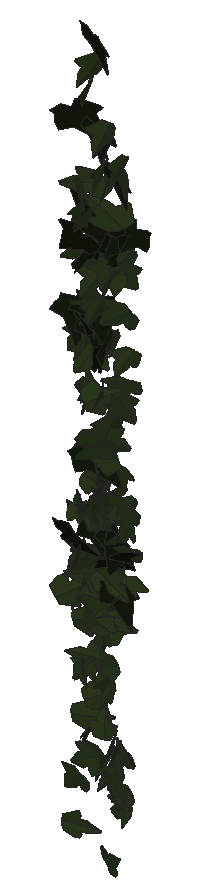
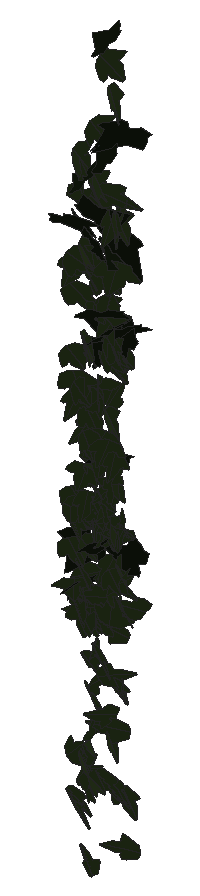
# SketchUp Ruby script. Lengths in inches.
U = 1.inch
M = Sketchup.active_model
def pt(a) = Geom::Point3d.new(a.map { |v| v * U })
def face(e, loops, mat)
  f = e.add_face(loops[0].map { |a| pt(a) })
  loops[1..].each { |l| e.add_face(l.map { |a| pt(a) }).erase! }
  f.material = f.back_material = mat if mat
  f
end
# faces: each face lists its corners as indices into pts; further lists are holes
def faces(e, pts, list, mat = nil) = list.each { |f| face(e, (f[0].is_a?(Array) ? f : [f]).map { |l| l.map { |i| pts[i] } }, mat) }
# xy, xz, yz: faces in a plane at the given z, y or x. An outline is a flat list of corners, or four numbers for a rectangle; further outlines are holes
def ring(l) = l.size == 4 ? [[l[0], l[1]], [l[2], l[1]], [l[2], l[3]], [l[0], l[3]]] : l.each_slice(2).to_a
def flat(e, list, mat, &to3) = list.each { |f| face(e, (f[0].is_a?(Array) ? f : [f]).map { |l| ring(l).map { |u, v| to3.(u, v) } }, mat) }
def xy(e, z, list, mat = nil) = flat(e, list, mat) { |x, y| [x, y, z] }
def xz(e, y, list, mat = nil) = flat(e, list, mat) { |x, z| [x, y, z] }
def yz(e, x, list, mat = nil) = flat(e, list, mat) { |y, z| [x, y, z] }
def lines(e, pts, list) = list.each { |a, b| e.add_line(pt(pts[a]), pt(pts[b])) }
# prism: a flat outline (further loops are holes) pulled along v
def prism(e, loops, v, mat = nil)
  f = face(e, loops, mat); d = Geom::Vector3d.new(v.map { |x| x * U })
  f.pushpull(f.normal.samedirection?(d) ? d.length : -d.length)
end
def box(e, o, s, mat = nil) = prism(e, [[o, [o[0] + s[0], o[1], o[2]], [o[0] + s[0], o[1] + s[1], o[2]], [o[0], o[1] + s[1], o[2]]]], [0, 0, s[2]], mat)
def at(x, y, z, deg = 0) = Geom::Transformation.translation(pt([x, y, z])) * Geom::Transformation.rotation(ORIGIN, Z_AXIS, deg.degrees)
def axes(o, x, y, z) = Geom::Transformation.new([*x, 0, *y, 0, *z, 0, *pt(o).to_a, 1])
def part(name) = M.definitions.add(name)
# library, detail: a bought-in or finely detailed component or shape, given as its bounding box
def library(name, o, s) = part(name).tap { |d| box(d.entities, o, s) }
def detail(e, o, s) = box(e.add_group.entities, o, s)
def put(e, d, t, mat = nil) = e.add_instance(d, t).tap { |i| i.material = mat if mat }
def group(e, t, mat = nil) = e.add_group.tap { |g| g.transformation = t; g.material = mat if mat }.entities
root = M.entities
M.materials.add("1026 AP 7946 SUNNY SIDE UP").color = [254, 231, 186]
M.materials.add("efeu1").color = [18, 25, 13]
M.materials.add("efeu2").color = [43, 57, 29]
c1 = part("ivyleaf_10")
p = [[0,0.5,-0.03],[-0.0625,2.02,-0.43],[-0.19,2.01,-0.46],[-0.54,1.05,-0.29],[-0.52,0.625,-0.18],[-0.83,0.76,-0.28],
  [-1.16,0.64,-0.33],[-1.15,0.33,-0.24],[-0.77,-0.39,0.02],[-0.3,-0.51,0.16],[0.04,-0.48,0.23],[-0.02,2.01,-0.4375],
  [-0.06,2.01,-0.43],[0.04,-0.49,0.23],[0.67,-0.49,0.14],[1.38,0.36,-0.2],[1.375,0.51,-0.24],[0.81,0.65,-0.19],
  [0.62,0.59,-0.15],[0.6,1.09,-0.28],[0.5,1.23,-0.31]]
faces(c1.entities,p,[[0,1,2,3,4,5,6,7,8,9,10],[11,12,0,13,14,15,16,17,18,19,20]],"efeu2")
c2 = part("ivyleaf_9")
p = [[1.54,2.16,1.25],[1.36,2.04,1.19],[-0.21,0.99,0.68],[-0.71,1.11,0.82],[-0.85,0.86,0.67],[-0.8,0.17,0.21],
  [-0.9,-0.01,0.1],[-0.67,-0.16,-0.02],[-0.08,-0.08,-0.05],[-0.03,-0.6,-0.4],[0.65,-0.88,-0.66],[0.83,-0.6,-0.49],
  [1.29,-0.42,-0.43],[1.8125,-0.07,-0.26],[1.21,0.44,0.15]]
faces(c2.entities,p,[[0,1,2,3,4,5,6,7,8,9,10,11,12,13,14]],"efeu1")
put(root,c1,axes([103.61,212.21,251.89],[-0.27089,0.03571,0.13207],[-0.20428,-0.00122,-0.1798],[-0.04391,-0.21462,0.02171]),"1026 AP 7946 SUNNY SIDE UP")
put(root,c1,axes([103.41,212.46,256.41],[-0.01976,-0.0299,0.20715],[0.11354,-0.18916,-0.02541],[0.29909,0.06983,0.02333]),"1026 AP 7946 SUNNY SIDE UP")
put(root,c2,axes([103.42,212.48,261.66],[-0.15715,-0.22456,-0.02631],[0.03236,0.01737,-0.25284],[0.35368,-0.10137,0.01144]),"1026 AP 7946 SUNNY SIDE UP")
put(root,c2,axes([103.32,212.4375,265.83],[-0.04557,-0.10489,-0.2458],[0.10836,0.22782,-0.11074],[0.39435,-0.07472,0.00202]),"1026 AP 7946 SUNNY SIDE UP")
put(root,c1,axes([103.59,212.45,261.22],[-0.1334,-0.17505,0.12633],[-0.05609,-0.11957,-0.20034],[0.33227,-0.09047,0.0169]),"1026 AP 7946 SUNNY SIDE UP")
put(root,c1,axes([103.43,212.65,258.53],[0.02494,-0.08582,0.20176],[0.14177,-0.17592,-0.08775],[0.30564,0.08861,0.02424]),"1026 AP 7946 SUNNY SIDE UP")
put(root,c2,axes([103.7,212.21,263.39],[0.16186,0.04053,-0.2429],[-0.35017,-0.07823,-0.11436],[-0.13841,0.24531,0.00528]),"1026 AP 7946 SUNNY SIDE UP")
put(root,c2,axes([103.22,212.32,256.83],[0.1703,-0.08723,0.20732],[0.20863,-0.15336,-0.14259],[0.27553,0.17004,-0.02018]),"1026 AP 7946 SUNNY SIDE UP")
put(root,c1,axes([103.45,212.41,255.82],[0.21725,-0.13904,0.11243],[0.10022,-0.09107,-0.20175],[0.26006,0.15125,-0.01617]),"1026 AP 7946 SUNNY SIDE UP")
put(root,c1,axes([103.5625,212.41,263.875],[0.01779,-0.23922,0.05053],[0.00255,-0.05039,-0.24701],[0.3844,0.0114,-0.0007]),"1026 AP 7946 SUNNY SIDE UP")
put(root,c1,axes([103.33,212.11,255.72],[0.14201,0.05417,-0.23523],[0.27143,0.15089,0.10795],[0.25066,-0.19408,0.01637]),"1026 AP 7946 SUNNY SIDE UP")
put(root,c1,axes([103.48,212.625,257.33],[0.0058,-0.07142,-0.19984],[0.01406,-0.19337,0.07255],[-0.32413,-0.00966,-0.00043]),"1026 AP 7946 SUNNY SIDE UP")
put(root,c1,axes([103.55,212.53,258.38],[-0.28661,0.09379,-0.01114],[0.00341,-0.0205,-0.21055],[-0.14851,-0.18147,0.01667]),"1026 AP 7946 SUNNY SIDE UP")
put(root,c1,axes([103.79,212.53,264.39],[0.16776,-0.0179,-0.23952],[-0.36435,-0.03577,-0.10696],[-0.03961,0.2532,-0.03052]),"1026 AP 7946 SUNNY SIDE UP")
put(root,c1,axes([103.47,212.4375,257.42],[0.18217,0.16732,0.0433],[0.0408,0.03199,-0.20945],[-0.26782,0.11869,-0.00246]),"1026 AP 7946 SUNNY SIDE UP")
put(root,c1,axes([103.71,212.49,252.23],[0.21608,-0.11136,-0.16322],[-0.21478,0.08089,-0.18087],[0.21472,0.19298,-0.01667]),"1026 AP 7946 SUNNY SIDE UP")
put(root,c1,axes([103.6,212.5625,256.54],[-0.12165,-0.17288,0.0748],[0.00088,-0.0798,-0.19298],[0.29544,-0.07094,0.03137]),"1026 AP 7946 SUNNY SIDE UP")
put(root,c1,axes([103.57,212.48,262.87],[-0.31656,-0.14651,-0.05002],[0.07939,0.01146,-0.2556],[0.2289,-0.20658,0.01948]),"1026 AP 7946 SUNNY SIDE UP")
put(root,c2,axes([103.34,212.44,261.35],[0.05466,-0.05707,0.26462],[0.13403,-0.24302,-0.06884],[0.39195,0.09106,-0.01336]),"1026 AP 7946 SUNNY SIDE UP")
put(root,c1,axes([103.83,212.31,257.33],[-0.05493,0.01768,-0.23778],[-0.29981,0.13034,0.04076],[0.20667,0.19378,-0.00407]),"1026 AP 7946 SUNNY SIDE UP")
put(root,c1,axes([103.48,212.39,264.24],[-0.13911,0.15671,-0.1847],[0.10801,-0.16733,-0.18565],[-0.35961,-0.11088,0.01569]),"1026 AP 7946 SUNNY SIDE UP")
put(root,c1,axes([103.53,212.39,256.65],[0.13148,-0.15203,0.1541],[0.09992,-0.13659,-0.17937],[0.32113,0.10475,-0.00728]),"1026 AP 7946 SUNNY SIDE UP")
put(root,c1,axes([103.41,212.44,257.58],[0.0799,-0.05103,0.19479],[0.24753,-0.10607,-0.07358],[0.18394,0.16491,0.0144]),"1026 AP 7946 SUNNY SIDE UP")
put(root,c1,axes([103.61,212.46,258.91],[-0.10047,-0.1749,-0.09713],[0.05897,0.08558,-0.19125],[0.30607,-0.0739,0.00497]),"1026 AP 7946 SUNNY SIDE UP")
put(root,c1,axes([103.63,212.59,259.85],[0.06703,-0.21488,0.03634],[0.00113,-0.03705,-0.2258],[0.34271,0.04215,-0.00636]),"1026 AP 7946 SUNNY SIDE UP")
put(root,c1,axes([103.38,212.26,250.8],[0.00055,0.01424,0.21153],[0.27157,0.11152,-0.00762],[-0.1758,0.17231,-0.01111]),"1026 AP 7946 SUNNY SIDE UP")
put(root,c1,axes([103.64,212.41,263.86],[0.19636,-0.18165,-0.1106],[-0.0115,0.11981,-0.21902],[0.33076,0.112,0.05804]),"1026 AP 7946 SUNNY SIDE UP")
put(root,c1,axes([103.67,212.5,255.59],[-0.33341,-0.03051,-0.01818],[-0.03117,0.01551,0.21999],[-0.04566,0.21219,-0.01742]),"1026 AP 7946 SUNNY SIDE UP")
put(root,c1,axes([103.79,212.48,254.35],[0.04297,0.05696,0.19953],[-0.17276,-0.15938,0.06343],[0.26573,-0.11283,0.00898]),"1026 AP 7946 SUNNY SIDE UP")
put(root,c1,axes([103.7,212.49,261.08],[-0.04657,-0.19853,0.13565],[-0.02194,-0.13215,-0.2075],[0.37493,-0.0324,0.00471]),"1026 AP 7946 SUNNY SIDE UP")
put(root,c1,axes([103.67,212.45,266.45],[0.07942,-0.2511,-0.02711],[-0.00605,0.02462,-0.26372],[0.39673,0.05064,0.0014]),"1026 AP 7946 SUNNY SIDE UP")
put(root,c1,axes([103.71,212.36,254.23],[0.26888,-0.09045,-0.06429],[-0.09491,0.018,-0.19882],[0.14384,0.18096,-0.01102]),"1026 AP 7946 SUNNY SIDE UP")
put(root,c1,axes([103.85,212.49,252.25],[0.17274,-0.10111,-0.19148],[-0.23638,0.10917,-0.15254],[0.233,0.1857,-0.01279]),"1026 AP 7946 SUNNY SIDE UP")
put(root,c1,axes([103.48,212.39,254.14],[0.10128,-0.04643,0.21667],[0.27428,-0.11799,-0.08246],[0.19935,0.18593,0.00337]),"1026 AP 7946 SUNNY SIDE UP")
put(root,c1,axes([103.9,212.28,256.24],[0.15765,-0.04672,-0.2011],[-0.30141,0.04145,-0.11155],[0.09225,0.21526,-0.0208]),"1026 AP 7946 SUNNY SIDE UP")
put(root,c1,axes([103.73,212.4375,261.38],[0.24024,-0.1706,-0.04919],[-0.0443,0.03756,-0.23567],[0.2746,0.15531,0.00501]),"1026 AP 7946 SUNNY SIDE UP")
put(root,c1,axes([103.69,212.43,260.05],[-0.04311,0.13514,0.20024],[0.08955,-0.18536,0.14052],[0.36029,0.06224,-0.01097]),"1026 AP 7946 SUNNY SIDE UP")
put(root,c1,axes([103.65,212.51,256.11],[0.01373,-0.04375,0.21633],[0.13983,-0.19079,-0.04582],[0.30735,0.08875,0.01118]),"1026 AP 7946 SUNNY SIDE UP")
put(root,c2,axes([103.87,212.15,262.97],[-0.22621,0.11335,-0.18737],[-0.19582,0.13501,0.18828],[0.2753,0.18917,-0.02004]),"1026 AP 7946 SUNNY SIDE UP")
put(root,c1,axes([103.71,212.5,261.36],[-0.01107,-0.17117,0.17476],[0.10213,-0.16574,-0.16952],[0.36603,0.04107,0.05259]),"1026 AP 7946 SUNNY SIDE UP")
put(root,c1,axes([103.9375,212.45,257.85],[-0.04535,0.04392,-0.20433],[-0.20651,0.14913,0.0545],[0.2442,0.13427,0.00814]),"1026 AP 7946 SUNNY SIDE UP")
put(root,c1,axes([103.76,212.32,263.77],[-0.07787,-0.20824,-0.14961],[0.07406,0.13663,-0.21937],[0.39118,-0.06732,0.01175]),"1026 AP 7946 SUNNY SIDE UP")
put(root,c2,axes([103.59,212.74,265.19],[0.04774,-0.17271,0.19226],[0.05207,-0.18466,-0.18174],[0.39757,0.04493,0.00072]),"1026 AP 7946 SUNNY SIDE UP")
put(root,c1,axes([103.84,212.46,261.79],[-0.32319,-0.10845,-0.05212],[-0.08072,-0.00957,0.23885],[-0.16953,0.21131,-0.01437]),"1026 AP 7946 SUNNY SIDE UP")
put(root,c1,axes([103.8125,212.37,260.9],[0.38473,-0.03452,-0.07064],[-0.11174,-0.01692,-0.25328],[0.04494,0.25349,-0.02501]),"1026 AP 7946 SUNNY SIDE UP")
put(root,c1,axes([103.83,212.3,252.99],[0.06254,-0.20851,-0.01696],[-0.01359,0.0139,-0.21851],[0.32846,0.04028,-0.00581]),"1026 AP 7946 SUNNY SIDE UP")
put(root,c1,axes([103.87,212.39,267.03],[-0.06527,-0.20567,0.16384],[-0.00571,-0.16175,-0.21584],[0.40988,-0.035,0.02308]),"1026 AP 7946 SUNNY SIDE UP")
put(root,c1,axes([103.85,212.45,257.18],[0.01619,0.2023,-0.07831],[-0.00197,0.07731,0.20907],[0.34045,-0.00917,0.00494]),"1026 AP 7946 SUNNY SIDE UP")
put(root,c1,axes([103.74,212.53,261.64],[-0.25801,0.11085,-0.11509],[0.09552,-0.10523,-0.19897],[-0.22906,-0.16874,0.04667]),"1026 AP 7946 SUNNY SIDE UP")
put(root,c1,axes([103.79,212.46,259.12],[-0.22339,-0.14035,-0.0661],[0.09909,0.02568,-0.20399],[0.22093,-0.15343,0.02465]),"1026 AP 7946 SUNNY SIDE UP")
put(root,c1,axes([103.875,212.27,257.67],[0.04457,-0.01716,0.25676],[-0.13336,0.23538,0.028],[-0.36966,-0.08699,0.02086]),"1026 AP 7946 SUNNY SIDE UP")
put(root,c1,axes([104.02,212.53,257.77],[-0.26313,0.01264,0.14209],[-0.21765,-0.01313,-0.17195],[-0.00217,-0.21641,0.01745]),"1026 AP 7946 SUNNY SIDE UP")
put(root,c1,axes([103.74,212.47,257.3125],[-0.26734,0.04343,-0.10572],[0.14529,-0.05048,-0.17958],[-0.09857,-0.1922,0.02202]),"1026 AP 7946 SUNNY SIDE UP")
put(root,c1,axes([103.78,212.29,258.23],[0.05838,0.12281,0.1845],[0.02306,0.17916,-0.12915],[-0.33977,0.03326,0.02294]),"1026 AP 7946 SUNNY SIDE UP")
put(root,c1,axes([103.875,212.61,264.65],[0.05749,-0.21899,0.0934],[0.04018,-0.08883,-0.22902],[0.37127,0.04352,0.01032]),"1026 AP 7946 SUNNY SIDE UP")
put(root,c2,axes([103.76,212.68,265.49],[-0.01316,-0.22886,0.09105],[-0.00167,-0.0897,-0.23644],[0.3865,-0.00818,0.00208]),"1026 AP 7946 SUNNY SIDE UP")
put(root,c1,axes([103.84,212.25,256.59],[-0.11819,-0.16243,-0.14014],[0.10193,0.11876,-0.18354],[0.31619,-0.099,0.00679]),"1026 AP 7946 SUNNY SIDE UP")
put(root,c1,axes([103.95,212.42,262.53],[-0.14283,-0.15696,0.17181],[-0.02524,-0.17552,-0.17926],[0.36025,-0.07453,0.05556]),"1026 AP 7946 SUNNY SIDE UP")
put(root,c1,axes([103.63,212.26,255.1875],[0.08001,-0.02034,-0.20436],[0.31146,-0.01741,0.05411],[-0.03457,-0.20394,0.01455]),"1026 AP 7946 SUNNY SIDE UP")
put(root,c1,axes([103.98,212.5,254.83],[0.186,-0.17549,-0.10046],[-0.10694,0.07024,-0.21702],[0.29621,0.13555,-0.01527]),"1026 AP 7946 SUNNY SIDE UP")
put(root,c1,axes([103.64,212.25,253.19],[0.04221,-0.01564,-0.22816],[0.33664,0.06058,0.02269],[0.09195,-0.21462,0.02167]),"1026 AP 7946 SUNNY SIDE UP")
put(root,c1,axes([103.76,212.38,253.54],[0.07049,0.00486,-0.21577],[0.20678,0.16611,0.03393],[0.25649,-0.13526,0.03194]),"1026 AP 7946 SUNNY SIDE UP")
put(root,c2,axes([104.16,212.3,263.6],[0.06619,0.02951,0.27735],[-0.32819,0.17689,0.01469],[-0.27096,-0.20705,0.04996]),"1026 AP 7946 SUNNY SIDE UP")
put(root,c2,axes([103.84,212.55,261.88],[-0.18535,-0.20665,-0.09579],[0.08706,0.07401,-0.24441],[0.34473,-0.1298,0.01022]),"1026 AP 7946 SUNNY SIDE UP")
put(root,c2,axes([103.82,212.5,261.41],[-0.02206,-0.25299,0.00991],[0.0049,-0.01125,-0.26107],[0.39815,-0.01388,0.00376]),"1026 AP 7946 SUNNY SIDE UP")
put(root,c1,axes([103.91,212.41,257.82],[-0.03369,-0.05896,-0.21352],[-0.01263,-0.20759,0.06058],[-0.33809,0.01363,0.01902]),"1026 AP 7946 SUNNY SIDE UP")
put(root,c1,axes([103.98,212.34,261.94],[-0.07476,-0.20053,0.09993],[0.01784,-0.10238,-0.21045],[0.3506,-0.03755,0.03202]),"1026 AP 7946 SUNNY SIDE UP")
put(root,c2,axes([103.76,212.47,267.49],[0.10083,-0.21718,0.13469],[0.05389,-0.12748,-0.23401],[0.39595,0.07265,-0.00245]),"1026 AP 7946 SUNNY SIDE UP")
put(root,c2,axes([103.85,212.57,257.14],[-0.0429,-0.24982,-0.04878],[0.02212,0.04464,-0.25847],[0.39879,-0.02935,0.00909]),"1026 AP 7946 SUNNY SIDE UP")
put(root,c1,axes([104,212.6,252.2],[0.06645,-0.16425,0.11897],[0.03098,-0.11501,-0.17521],[0.31504,0.04595,-0.00786]),"1026 AP 7946 SUNNY SIDE UP")
put(root,c1,axes([103.98,212.61,264.47],[0.18142,-0.18989,0.08964],[0.0652,-0.07786,-0.22931],[0.32263,0.12252,-0.00407]),"1026 AP 7946 SUNNY SIDE UP")
put(root,c1,axes([104.03,212.3,258.89],[-0.23216,-0.19963,-0.04561],[0.05844,0.02608,-0.25523],[0.31578,-0.15159,0.0137]),"1026 AP 7946 SUNNY SIDE UP")
put(root,c2,axes([103.83,212.28,258.82],[0.01407,-0.16686,-0.18717],[0.10129,0.17613,-0.1632],[0.37329,-0.0415,0.05134]),"1026 AP 7946 SUNNY SIDE UP")
put(root,c1,axes([104.26,212.32,258.77],[0.08403,0.02118,-0.23381],[-0.35118,-0.04238,-0.05846],[-0.07264,0.2294,0.01219]),"1026 AP 7946 SUNNY SIDE UP")
put(root,c1,axes([104.1,212.2,258.49],[-0.1848,0.15924,0.06997],[-0.09269,0.03923,-0.20229],[-0.25536,-0.12948,0.02279]),"1026 AP 7946 SUNNY SIDE UP")
put(root,c1,axes([104.02,212.3,259.17],[-0.29381,-0.10376,-0.0706],[0.10598,0.01817,-0.21945],[0.1637,-0.19799,0.01537]),"1026 AP 7946 SUNNY SIDE UP")
put(root,c1,axes([104.09,212.375,254.93],[0.04514,-0.06503,-0.21156],[-0.00527,0.20665,-0.06681],[0.33812,0.0119,0.0272]),"1026 AP 7946 SUNNY SIDE UP")
put(root,c1,axes([104.07,212.45,265.64],[-0.0872,-0.20808,0.16004],[0.06613,-0.1651,-0.21171],[0.40404,-0.01788,0.06919]),"1026 AP 7946 SUNNY SIDE UP")
put(root,c1,axes([104.13,212.24,260.21],[0.0631,-0.19806,-0.13296],[-0.00717,0.12911,-0.20661],[0.37069,0.03621,0.01864]),"1026 AP 7946 SUNNY SIDE UP")
put(root,c2,axes([104.11,212.2,260.8],[-0.02451,-0.08523,0.25076],[0.16604,0.2209,0.08777],[-0.37077,0.10456,0.02273]),"1026 AP 7946 SUNNY SIDE UP")
put(root,c1,axes([103.82,212.42,255.39],[0.00545,0.01795,0.25613],[0.38188,-0.05579,0.00033],[0.08757,0.2422,-0.0174]),"1026 AP 7946 SUNNY SIDE UP")
put(root,c1,axes([104.01,212.47,260.02],[-0.22795,0.12471,-0.12201],[0.13042,-0.08604,-0.19727],[-0.23778,-0.16675,0.00876]),"1026 AP 7946 SUNNY SIDE UP")
put(root,c1,axes([104.11,212.6,261.15],[0.12251,-0.20348,0.05312],[0.0339,-0.0482,-0.22472],[0.32877,0.08079,0.00337]),"1026 AP 7946 SUNNY SIDE UP")
put(root,c1,axes([104.17,212.34,257.37],[0.12838,-0.1512,-0.14437],[-0.02677,0.14437,-0.1709],[0.32213,0.07226,0.04333]),"1026 AP 7946 SUNNY SIDE UP")
put(root,c1,axes([104.09,212.45,254.07],[-0.04938,-0.0022,0.21988],[0.10153,-0.20574,0.0064],[0.31992,0.06496,0.03191]),"1026 AP 7946 SUNNY SIDE UP")
put(root,c1,axes([104.18,212.57,259.2],[-0.03607,-0.21362,0.02165],[-0.00022,-0.02234,-0.22146],[0.33771,-0.02283,0.00217]),"1026 AP 7946 SUNNY SIDE UP")
put(root,c1,axes([104.33,212.27,257.51],[0.10388,0.02706,0.20723],[-0.28153,0.10708,0.0464],[-0.1498,-0.18248,0.0565]),"1026 AP 7946 SUNNY SIDE UP")
put(root,c1,axes([104.39,212.35,262.74],[0.19748,-0.07828,-0.22195],[-0.32736,0.06265,-0.14842],[0.14925,0.24099,-0.03186]),"1026 AP 7946 SUNNY SIDE UP")
put(root,c1,axes([104.13,212.45,258.27],[0.22121,-0.1793,0.06112],[0.04596,-0.0537,-0.23488],[0.2939,0.14335,-0.00927]),"1026 AP 7946 SUNNY SIDE UP")
put(root,c1,axes([104.18,212.26,253],[0.07611,0.21636,-0.09263],[0.02251,0.09017,0.22887],[0.36847,-0.0502,0.00515]),"1026 AP 7946 SUNNY SIDE UP")
put(root,c1,axes([104.2,212.42,253.86],[0.23346,-0.17833,-0.00292],[-0.01773,-0.00703,-0.23871],[0.27986,0.14832,-0.01269]),"1026 AP 7946 SUNNY SIDE UP")
put(root,c1,axes([104.17,212.29,258.31],[0.10221,-0.1525,0.15227],[-0.05777,0.14508,0.17071],[-0.32987,-0.07266,0.01728]),"1026 AP 7946 SUNNY SIDE UP")
put(root,c1,axes([104.25,212.4375,262.78],[-0.20111,-0.18594,0.08559],[-0.02008,-0.0918,-0.22955],[0.32028,-0.12251,0.03935]),"1026 AP 7946 SUNNY SIDE UP")
put(root,c1,axes([104.03,212.2,255.21],[-0.20531,-0.07012,0.16936],[0.20657,0.10111,0.15214],[-0.19139,0.18435,-0.01747]),"1026 AP 7946 SUNNY SIDE UP")
put(root,c1,axes([104.1875,212.64,263.15],[0.1064,-0.21047,0.08013],[0.03151,-0.0765,-0.22816],[0.35207,0.07045,-0.00379]),"1026 AP 7946 SUNNY SIDE UP")
put(root,c1,axes([104,212.12,260.04],[0.08188,0.03342,-0.25697],[0.274,0.17927,0.06322],[0.28593,-0.18136,0.013]),"1026 AP 7946 SUNNY SIDE UP")
put(root,c1,axes([104.2,212.52,257.9375],[-0.13869,-0.18093,-0.08338],[0.05905,0.07058,-0.20693],[0.30535,-0.09583,0.00215]),"1026 AP 7946 SUNNY SIDE UP")
put(root,c1,axes([104.26,212.53,261.21],[0.11305,-0.20668,-0.07183],[-0.03327,0.06522,-0.22505],[0.34077,0.07493,0.00186]),"1026 AP 7946 SUNNY SIDE UP")
put(root,c1,axes([104.39,212.29,251.79],[0.02902,0.02171,0.21274],[-0.26351,0.12376,0.00275],[-0.19245,-0.16619,0.02831]),"1026 AP 7946 SUNNY SIDE UP")
put(root,c2,axes([104.05,212.45,263.03],[-0.06236,0.12768,0.22277],[0.13112,-0.19903,0.13611],[0.37142,0.0917,-0.01065]),"1026 AP 7946 SUNNY SIDE UP")
put(root,c1,axes([103.96,212.22,255.81],[-0.06502,-0.04223,-0.24335],[0.3696,0.03991,-0.04956],[0.07406,-0.23623,0.03366]),"1026 AP 7946 SUNNY SIDE UP")
put(root,c1,axes([104.24,212.36,252.53],[0.11673,-0.14653,0.1252],[-0.08336,0.1103,0.16986],[-0.28837,-0.0912,0.00158]),"1026 AP 7946 SUNNY SIDE UP")
put(root,c1,axes([104.37,212.28,254.46],[0.17102,-0.10368,-0.15033],[-0.18878,0.08348,-0.15342],[0.20776,0.16119,-0.01566]),"1026 AP 7946 SUNNY SIDE UP")
put(root,c1,axes([104.28,212.42,252.11],[-0.05581,-0.14902,0.1393],[-0.00925,-0.13733,-0.15733],[0.31716,-0.03022,0.01992]),"1026 AP 7946 SUNNY SIDE UP")
put(root,c1,axes([104.27,212.49,256.96],[0.01026,-0.19177,0.09446],[0.00746,-0.09267,-0.19821],[0.33488,0.00794,0.00152]),"1026 AP 7946 SUNNY SIDE UP")
put(root,c1,axes([104.26,212.57,252.55],[0.08916,-0.1989,0.01521],[-0.00181,-0.01685,-0.21308],[0.31374,0.05643,-0.00556]),"1026 AP 7946 SUNNY SIDE UP")
put(root,c1,axes([104.31,212.34,259.6],[-0.11168,-0.22167,0.06407],[-0.01538,-0.06344,-0.23996],[0.36223,-0.07104,0.00956]),"1026 AP 7946 SUNNY SIDE UP")
put(root,c1,axes([104.25,212.56,258.49],[-0.31471,0.05705,-0.02728],[0.03062,-0.02889,-0.21334],[-0.09427,-0.19986,0.02176]),"1026 AP 7946 SUNNY SIDE UP")
put(root,c1,axes([104.22,212.42,262.58],[0.16579,-0.18874,0.10711],[0.05775,-0.09952,-0.22278],[0.33469,0.11067,-0.01461]),"1026 AP 7946 SUNNY SIDE UP")
put(root,c1,axes([104.46,212.28,263.91],[0.23887,0.13698,0.19223],[-0.24376,-0.10429,0.20916],[0.26897,-0.21617,0.01884]),"1026 AP 7946 SUNNY SIDE UP")
put(root,c1,axes([104.1,212.57,255.31],[-0.09927,0.01057,0.20062],[0.2674,-0.09708,0.06168],[0.14991,0.18017,0.02283]),"1026 AP 7946 SUNNY SIDE UP")
put(root,c1,axes([104.31,212.64,260.23],[-0.02349,-0.19371,0.10564],[0.0104,-0.10423,-0.20032],[0.34529,-0.01004,0.01322]),"1026 AP 7946 SUNNY SIDE UP")
put(root,c2,axes([104.12,212.6875,264.61],[0.07586,-0.21581,0.11103],[0.03441,-0.1068,-0.22843],[0.37861,0.05295,-0.00149]),"1026 AP 7946 SUNNY SIDE UP")
put(root,c1,axes([104.35,212.73,262.96],[-0.09176,-0.17197,0.20039],[-0.00054,-0.2003,-0.18279],[0.40941,-0.03881,0.04467]),"1026 AP 7946 SUNNY SIDE UP")
put(root,c1,axes([104.29,212.56,256.43],[0.24501,-0.13907,0.02749],[0.01817,-0.02822,-0.21489],[0.22216,0.15568,-0.01273]),"1026 AP 7946 SUNNY SIDE UP")
put(root,c1,axes([104.39,212.54,257.66],[-0.12093,-0.16987,0.09869],[-0.05103,-0.09144,-0.19249],[0.30313,-0.08316,0.00697]),"1026 AP 7946 SUNNY SIDE UP")
put(root,c1,axes([104.41,212.41,252.39],[0.18364,-0.15341,-0.07406],[-0.09043,0.04512,-0.19757],[0.24997,0.12903,-0.01706]),"1026 AP 7946 SUNNY SIDE UP")
put(root,c1,axes([104.21,212.38,250.17],[-0.20654,0.07364,0.14341],[0.21143,-0.04088,0.15321],[0.12778,0.18667,-0.0217]),"1026 AP 7946 SUNNY SIDE UP")
put(root,c1,axes([104.43,212.18,255.08],[0.24262,-0.05446,0.13254],[-0.17845,0.06373,0.16797],[-0.1289,-0.19073,0.01694]),"1026 AP 7946 SUNNY SIDE UP")
put(root,c1,axes([104.4,212.31,255.39],[-0.33549,-0.06645,0.00765],[-0.00165,-0.02274,-0.22929],[0.10518,-0.21229,0.02079]),"1026 AP 7946 SUNNY SIDE UP")
put(root,c1,axes([104.46,212.5625,260.35],[-0.27839,-0.11995,0.05878],[-0.05739,-0.04865,-0.21971],[0.2013,-0.17975,0.01865]),"1026 AP 7946 SUNNY SIDE UP")
put(root,c2,axes([104.31,212.52,256.93],[-0.08438,-0.21874,0.1267],[-0.01439,-0.12524,-0.23199],[0.39528,-0.05126,0.0186]),"1026 AP 7946 SUNNY SIDE UP")
put(root,c1,axes([104.375,212.55,264.99],[0.04012,-0.22246,0.16299],[0.07616,-0.15397,-0.23015],[0.4236,0.04875,0.02594]),"1026 AP 7946 SUNNY SIDE UP")
put(root,c1,axes([104.6,212.4,257.8125],[-0.30539,0.00899,0.14912],[-0.22753,-0.02681,-0.19853],[0.01394,-0.2407,0.02626]),"1026 AP 7946 SUNNY SIDE UP")
put(root,c1,axes([104.55,212.49,251.68],[0.15943,-0.09076,-0.15931],[-0.20504,0.08375,-0.1387],[0.1925,0.16438,-0.01579]),"1026 AP 7946 SUNNY SIDE UP")
put(root,c1,axes([104.38,212.43,252.04],[-0.06698,0.14122,0.19774],[0.08097,-0.1841,0.15086],[0.36482,0.06679,0.00282]),"1026 AP 7946 SUNNY SIDE UP")
put(root,c1,axes([104.64,212.32,261.99],[-0.25649,-0.0235,0.17495],[-0.24366,-0.0805,-0.16515],[0.11582,-0.22139,0.04]),"1026 AP 7946 SUNNY SIDE UP")
put(root,c1,axes([104.23,212.62,255.49],[-0.0865,0.0535,0.21699],[0.2838,-0.1092,0.07662],[0.18949,0.18798,-0.01569]),"1026 AP 7946 SUNNY SIDE UP")
put(root,c1,axes([104.48,212.65,260.92],[-0.15382,-0.16027,0.12383],[-0.0105,-0.13204,-0.18634],[0.31569,-0.08249,0.05414]),"1026 AP 7946 SUNNY SIDE UP")
put(root,c1,axes([104.2,212.24,256.28],[0.21068,0.07342,0.18005],[0.26254,0.05457,-0.15553],[-0.13987,0.21301,-0.02074]),"1026 AP 7946 SUNNY SIDE UP")
put(root,c1,axes([104.6,212.39,251.47],[0.14662,-0.13939,-0.18203],[-0.18304,0.13283,-0.17123],[0.30174,0.14831,-0.01541]),"1026 AP 7946 SUNNY SIDE UP")
put(root,c1,axes([104.48,212.28,255.94],[0.02695,-0.19306,-0.07087],[-0.00808,0.06751,-0.19928],[0.32159,0.01788,0.00093]),"1026 AP 7946 SUNNY SIDE UP")
put(root,c1,axes([104.39,212.17,259.29],[-0.09116,-0.15443,-0.20605],[0.15245,0.17494,-0.16782],[0.36574,-0.11141,0.01859]),"1026 AP 7946 SUNNY SIDE UP")
put(root,c1,axes([104.5,212.45,264.75],[0.23134,-0.17481,-0.10646],[-0.05212,0.10402,-0.2315],[0.31422,0.14595,0.03998]),"1026 AP 7946 SUNNY SIDE UP")
put(root,c1,axes([104.48,212.6875,257.74],[-0.02793,-0.12743,0.17405],[0.03638,-0.17042,-0.13036],[0.33167,0.00796,0.02896]),"1026 AP 7946 SUNNY SIDE UP")
put(root,c1,axes([104.59,212.51,256.83],[-0.21328,-0.14188,0.07844],[-0.06804,-0.06487,-0.20217],[0.2445,-0.14182,0.01217]),"1026 AP 7946 SUNNY SIDE UP")
put(root,c1,axes([104.64,212.42,252.45],[-0.22548,0.0948,-0.11874],[-0.13556,0.07877,0.17687],[0.19235,0.16664,-0.01454]),"1026 AP 7946 SUNNY SIDE UP")
put(root,c1,axes([104.45,212.47,259.94],[-0.14142,-0.20013,-0.11188],[0.12329,0.08113,-0.22277],[0.33523,-0.11426,0.03473]),"1026 AP 7946 SUNNY SIDE UP")
put(root,c2,axes([104.44,212.14,256.8],[0.22047,0.20139,0.06617],[0.07449,0.04377,-0.25217],[-0.32337,0.14739,-0.01298]),"1026 AP 7946 SUNNY SIDE UP")
put(root,c2,axes([104.62,212.63,263.63],[-0.34852,-0.10289,0.00705],[0.00318,-0.02192,-0.25096],[0.16218,-0.22068,0.02006]),"1026 AP 7946 SUNNY SIDE UP")
put(root,c1,axes([104.49,212.49,262.73],[-0.18062,-0.18254,-0.11403],[0.10057,0.08926,-0.22158],[0.31937,-0.13134,0.00528]),"1026 AP 7946 SUNNY SIDE UP")
put(root,c1,axes([104.46,212.57,256.12],[0.22443,0.17147,-0.01625],[-0.00275,-0.02031,-0.22964],[-0.27089,0.14227,-0.01113]),"1026 AP 7946 SUNNY SIDE UP")
put(root,c1,axes([104.38,212.24,255.38],[0.32727,0.0508,-0.11025],[0.15383,0.04932,0.21982],[0.10576,-0.22891,0.02143]),"1026 AP 7946 SUNNY SIDE UP")
put(root,c1,axes([104.55,212.49,257.4],[0.26575,-0.10737,-0.05139],[-0.04074,0.05022,-0.204],[0.18124,0.16873,0.02949]),"1026 AP 7946 SUNNY SIDE UP")
put(root,c2,axes([104.4,212.4,256.0625],[0.02339,-0.24576,-0.06655],[-0.00666,0.06307,-0.25327],[0.39895,0.01546,-0.00033]),"1026 AP 7946 SUNNY SIDE UP")
